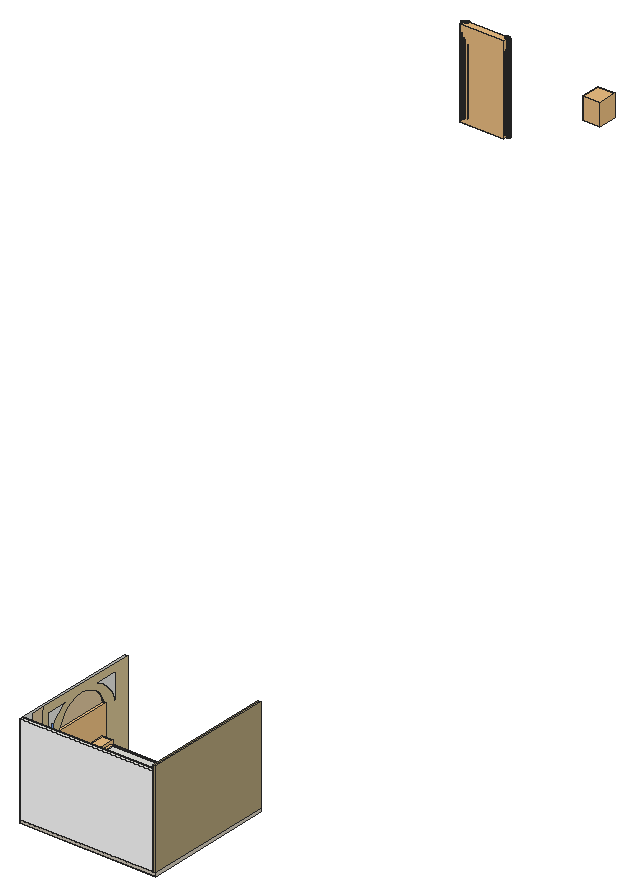
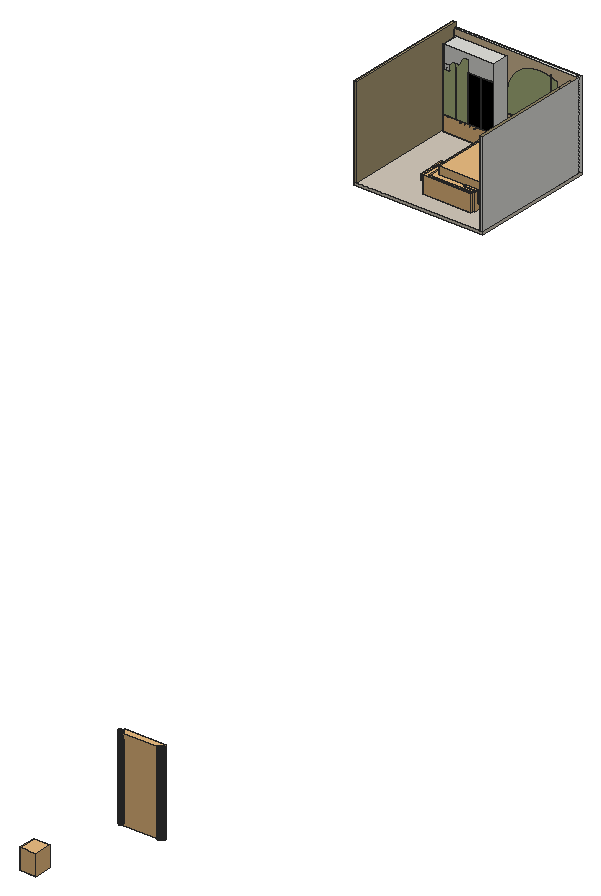
# SketchUp Ruby script. Lengths in inches.
U = 1.inch
M = Sketchup.active_model
def pt(a) = Geom::Point3d.new(a.map { |v| v * U })
def face(e, loops, mat)
  f = e.add_face(loops[0].map { |a| pt(a) })
  loops[1..].each { |l| e.add_face(l.map { |a| pt(a) }).erase! }
  f.material = f.back_material = mat if mat
  f
end
# faces: each face lists its corners as indices into pts; further lists are holes
def faces(e, pts, list, mat = nil) = list.each { |f| face(e, (f[0].is_a?(Array) ? f : [f]).map { |l| l.map { |i| pts[i] } }, mat) }
# xy, xz, yz: faces in a plane at the given z, y or x. An outline is a flat list of corners, or four numbers for a rectangle; further outlines are holes
def ring(l) = l.size == 4 ? [[l[0], l[1]], [l[2], l[1]], [l[2], l[3]], [l[0], l[3]]] : l.each_slice(2).to_a
def flat(e, list, mat, &to3) = list.each { |f| face(e, (f[0].is_a?(Array) ? f : [f]).map { |l| ring(l).map { |u, v| to3.(u, v) } }, mat) }
def xy(e, z, list, mat = nil) = flat(e, list, mat) { |x, y| [x, y, z] }
def xz(e, y, list, mat = nil) = flat(e, list, mat) { |x, z| [x, y, z] }
def yz(e, x, list, mat = nil) = flat(e, list, mat) { |y, z| [x, y, z] }
def lines(e, pts, list) = list.each { |a, b| e.add_line(pt(pts[a]), pt(pts[b])) }
# prism: a flat outline (further loops are holes) pulled along v
def prism(e, loops, v, mat = nil)
  f = face(e, loops, mat); d = Geom::Vector3d.new(v.map { |x| x * U })
  f.pushpull(f.normal.samedirection?(d) ? d.length : -d.length)
end
def box(e, o, s, mat = nil) = prism(e, [[o, [o[0] + s[0], o[1], o[2]], [o[0] + s[0], o[1] + s[1], o[2]], [o[0], o[1] + s[1], o[2]]]], [0, 0, s[2]], mat)
def at(x, y, z, deg = 0) = Geom::Transformation.translation(pt([x, y, z])) * Geom::Transformation.rotation(ORIGIN, Z_AXIS, deg.degrees)
def axes(o, x, y, z) = Geom::Transformation.new([*x, 0, *y, 0, *z, 0, *pt(o).to_a, 1])
def part(name) = M.definitions.add(name)
# library, detail: a bought-in or finely detailed component or shape, given as its bounding box
def library(name, o, s) = part(name).tap { |d| box(d.entities, o, s) }
def detail(e, o, s) = box(e.add_group.entities, o, s)
def put(e, d, t, mat = nil) = e.add_instance(d, t).tap { |i| i.material = mat if mat }
def group(e, t, mat = nil) = e.add_group.tap { |g| g.transformation = t; g.material = mat if mat }.entities
root = M.entities
M.materials.add("BACK Wall colour").color = [219, 194, 155]
M.materials.add("CREAM BOARD").color = [211, 192, 145]
M.materials.add("Emissive").color = [255, 225, 187]
M.materials.add("Emissive\#1").color = [255, 255, 255]
M.materials.add("Marble").color = [211, 202, 187]
M.materials.add("Material__1").color = [146, 146, 144]
M.materials.add("Material__10").color = [208, 163, 136]
M.materials.add("Material__11").color = [204, 203, 204]
M.materials.add("Material__2").color = [184, 175, 165]
M.materials.add("Material__3").color = [220, 221, 223]
M.materials.add("Material__4").color = [119, 115, 113]
M.materials.add("Material__5").color = [191, 184, 174]
M.materials.add("Material__6").color = [181, 176, 158]
M.materials.add("Material__8").color = [243, 243, 243]
M.materials.add("Material__9").color = [193, 193, 193]
M.materials.add("[Color A01]").color = [173, 157, 118]
M.materials.add("[Color M07]").color = [57, 57, 57]
M.materials.add("[Translucent Glass Blue]").color = [100, 149, 237]
M.materials["[Translucent Glass Blue]"].alpha = 0.5
M.materials.add("cubod").color = [174, 185, 130]
M.materials.add("mirror").color = [0, 0, 0]
M.materials.add("wire_1").color = [252, 248, 227]
M.materials.add("wire_2").color = [148, 176, 27]
M.materials.add("wire_3").color = [246, 240, 240]
M.materials.add("wire_4").color = [250, 248, 254]
M.materials.add("wire_5").color = [223, 86, 86]
M.materials.add("ไม้ระแนง").color = [255, 207, 170]
c1 = library("Group\#139",[0,-0.62,-0.17],[22.83,25.13,29.45])
c2 = part("Group\#298")
box(c2.entities,[1.18,0.2,0],[0.79,0.19,118.11])
c3 = part("Group\#129")
put(c3.entities,c2,at(1.68,1.9,0,-75.963))
put(c3.entities,c2,at(1.875,1.69,0,-18.991))
put(c3.entities,c2,at(1.72,1.81,0,-56.972))
put(c3.entities,c2,at(1.7,1.85,0,-66.468))
put(c3.entities,c2,at(2.26,1.99,0,94.13))
put(c3.entities,c2,at(1.92,1.68,0,-9.495))
put(c3.entities,c2,at(1.67,2,0,-94.954))
put(c3.entities,c2,at(1.79,1.74,0,-37.981))
put(c3.entities,c2,at(1.7,2.09,0,-113.944))
put(c3.entities,c2,at(1.83,1.71,0,-28.486))
put(c3.entities,c2,at(1.75,1.77,0,-47.477))
put(c3.entities,c2,at(1.68,2.04,0,-104.449))
put(c3.entities,c2,at(1.67,1.95,0,-85.458))
put(c3.entities,c2,at(2.26,1.94,0,84.634))
put(c3.entities,c2,at(1.97,1.67,0))
put(c3.entities,c2,at(2.1875,2.17,0,132.111))
put(c3.entities,c2,at(1.83,2.23,0,-151.926))
put(c3.entities,c2,at(1.75,2.17,0,-132.935))
put(c3.entities,c2,at(1.72,2.13,0,-123.44))
put(c3.entities,c2,at(2.07,2.25,0,160.597))
put(c3.entities,c2,at(2.24,2.09,0,113.12))
put(c3.entities,c2,at(1.92,2.26,0,-170.917))
put(c3.entities,c2,at(2.02,2.26,0,170.093))
put(c3.entities,c2,at(2.11,2.23,0,151.102))
put(c3.entities,c2,at(2.15,2.2,0,141.607))
put(c3.entities,c2,at(2.22,2.13,0,122.616))
put(c3.entities,c2,at(1.875,2.25,0,-161.421))
put(c3.entities,c2,at(2.26,2.04,0,103.625))
put(c3.entities,c2,at(1.79,2.2,0,-142.431))
put(c3.entities,c2,at(1.97,2.27,0,179.588))
put(c3.entities,c2,at(2.0625,1.69,0,18.167))
put(c3.entities,c2,at(2.18,1.77,0,46.653))
put(c3.entities,c2,at(2.25,1.89,0,75.139))
put(c3.entities,c2,at(2.15,1.73,0,37.157))
put(c3.entities,c2,at(2.01,1.68,0,8.671))
put(c3.entities,c2,at(1.92,1.68,0,-10.319))
put(c3.entities,c2,at(1.96,1.67,0,-0.824))
put(c3.entities,c2,at(2.21,1.81,0,56.148))
put(c3.entities,c2,at(1.87,1.69,0,-19.815))
put(c3.entities,c2,at(2.24,1.85,0,65.644))
put(c3.entities,c2,at(2.11,1.71,0,27.662))
c4 = library("Group\#135",[0,0,0],[59.06,10.24,118.11])
c5 = library("Group\#97",[220.84,467.58,-548.74],[526,430.5,273.26])
c6 = library("Group\#96",[16.29,461.76,-808.58],[654.47,563.24,342.1])
c7 = library("Group\#95",[26.77,467.46,-1024.34],[745.52,615.51,329.95])
c8 = library("Group\#94",[-756.47,467.51,-1025.0625],[743.88,650.18,302.68])
c9 = library("Group\#93",[-553.95,461.3125,-816.79],[663.59,570.86,267.16])
c10 = library("Group\#92",[-509.59,467.57,-586.51],[732.34,417.16,267.86])
c11 = library("Group\#91",[-1172.66,2.01,-321.31],[2325.11,593.39,1560.68])
c12 = library("Group\#90",[-1281.34,1.4,-240.6],[2502.68,574.48,1653.76])
c13 = library("Group\#89",[-1090.55,247.54,-372.01],[2133.07,362.54,526.23])
c14 = library("Group\#88",[-193.83,481.2,453.03],[613.57,176.39,387.44])
c15 = library("Group\#87",[-955.4375,-0.64,-1094.53],[1900,840.64,2180.25])
c16 = library("Group\#86",[-945.74,207.56,-988.65],[1854.67,255.51,2057.08])
c17 = library("Group\#85",[-22.63,147.2,1249.93],[883.21,192.64,509.1])
c18 = library("Group\#104",[189.08,342.22,1232.64],[352.42,17.32,353.57])
c19 = library("Group\#105",[41.45,326.8125,1372.4],[357.97,38.32,359.1])
c20 = library("Group\#106",[39.12,326.04,1373.29],[358.62,26.89,359.71])
c21 = library("Group\#98",[-1244.68,656.3,-867.46],[92.26,185.35,88.07])
c22 = library("Group\#99",[-1423.96,598.21,-801.8],[288.83,436.59,261.62])
c23 = library("Group\#100",[-1158.34,656.31,-821.02],[80.76,145.22,75.04])
c24 = library("Group\#101",[-1453.32,0.83,-981.3],[432.86,597.97,432.82])
c25 = library("Group\#102",[-1264.29,598.92,-883.28],[205.66,57.91,141.8])
c26 = library("Group\#103",[202.625,359.35,1362.02],[142.76,55.22,150.9])
c27 = part("bed")
g1 = group(c27.entities,at(-348.48,-2600.07,-0.46))
put(g1,c5,axes([1281.34,1759.03,0.64],[1,0,0],[0,0,1],[0,-1,0]),"Material__1")
put(g1,c6,axes([1281.34,1759.03,0.64],[1,0,0],[0,0,1],[0,-1,0]),"Material__2")
put(g1,c7,axes([1281.34,1759.03,0.64],[1,0,0],[0,0,1],[0,-1,0]),"Material__3")
put(g1,c8,axes([1281.34,1759.03,0.64],[1,0,0],[0,0,1],[0,-1,0]),"Material__2")
put(g1,c9,axes([1281.34,1759.03,0.64],[1,0,0],[0,0,1],[0,-1,0]),"Material__3")
put(g1,c10,axes([1281.34,1759.03,0.64],[1,0,0],[0,0,1],[0,-1,0]),"Material__4")
put(g1,c11,axes([1281.34,1759.03,0.64],[1,0,0],[0,0,1],[0,-1,0]),"Material__2")
put(g1,c12,axes([1281.34,1759.03,0.64],[1,0,0],[0,0,1],[0,-1,0]),"Material__4")
put(g1,c13,axes([1281.34,1759.03,0.64],[1,0,0],[0,0,1],[0,-1,0]),"Material__3")
put(g1,c14,axes([1281.34,1759.03,0.64],[1,0,0],[0,0,1],[0,-1,0]),"Material__5")
put(g1,c15,axes([1281.34,1759.03,0.64],[1,0,0],[0,0,1],[0,-1,0]),"Material__6")
put(g1,c16,axes([1281.34,1759.03,0.64],[1,0,0],[0,0,1],[0,-1,0]),"wire_1")
put(g1,c17,axes([1281.34,1759.03,0.64],[1,0,0],[0,0,1],[0,-1,0]),"Material__6")
g2 = group(g1,at(1281.34,1759.03,0.64),"Material__6")
p = [[51.41,-1680.01,120.74],[789.14,-1719.33,120.75],[51.38,-1719.36,120.79],[51.38,-1680.06,160.45],[788.85,-1679.65,121.17],[789.14,-1679.64,160.07],
  [788.85,-1718.96,160.45],[51.74,-1719.36,160.07]]
faces(g2,p,[[0,1,2],[3,0,2],[0,4,1],[0,3,5],[0,5,4],[6,2,1],[6,7,2],[3,2,7],
  [6,1,4],[6,4,5],[7,5,3],[7,6,5]],"[Color M07]")
g3 = group(g1,at(1281.34,1759.03,0.64),"Material__6")
p = [[788.42,-1678.8,120.79],[827.72,-1336.33,121.1],[827.72,-1678.5,120.76],[788.4,-1336.69,121.17],[788.38,-1336.73,160.09],[788.41,-1678.49,160.09],
  [828.07,-1678.51,160.45],[828.09,-1336.73,160.41]]
faces(g3,p,[[0,1,2],[0,3,1],[0,4,3],[0,5,4],[7,2,1],[7,6,2],[7,1,3],[7,3,4],
  [6,4,5],[6,7,4]],"[Color M07]")
faces(g3,p,[[5,0,2],[5,2,6]],"Material__6")
g4 = group(g1,at(1281.34,1759.03,0.64),"Material__6")
p = [[51.36,-1295.89,160.46],[51.45,-1335.18,120.84],[51.35,-1333.34,160.1],[52.33,-1335.21,158.6],[51.47,-1295.85,120.75],[789.16,-1335.14,120.79],
  [788.81,-1335.18,160.42],[789.15,-1295.51,120.8125],[788.78,-1295.48,160.09]]
faces(g4,p,[[0,1,2],[1,3,2],[4,5,1],[6,1,5],[6,3,1],[0,4,1],[6,7,8],[6,5,7],
  [4,7,5],[4,0,8],[4,8,7],[6,2,3],[2,6,8],[2,8,0]],"[Color M07]")
g5 = group(g1,at(1281.34,1759.03,0.64),"Material__6")
p = [[12.71,-1678.78,120.74],[12.34,-1336.83,160.45],[12.72,-1336.33,121.11],[12.71,-1678.52,160.09],[51.7,-1336.34,121.1],[52.03,-1678.85,120.78],
  [52.03,-1678.82,160.45],[52.06,-1336.72,160.4]]
faces(g5,p,[[0,1,2],[0,3,1],[0,4,5],[0,2,4],[3,0,5],[3,5,6],[7,5,4],[7,6,5],
  [7,2,1],[7,4,2],[6,1,3],[6,7,1]],"[Color M07]")
g6 = group(g1,at(1281.34,1759.03,0.64),"Material__6")
xy(g6,160.97,[[12.77,-1334.88,51.14,-1295.51,11.77,-1296.13],[12.77,-1334.88,51.14,-1334.51,51.14,-1295.51]],"[Color M07]")
p = [[11.77,-1296.13,160.97],[11.86,-1295.16,1.14],[11.8,-1334.85,1.21],[45.68,-1334.49,1.53],[45.32,-1295.17,1.54],[51.14,-1295.51,160.97],
  [12.77,-1334.88,160.97],[51.14,-1334.51,160.97]]
faces(g6,p,[[0,1,2],[3,2,1],[3,1,4],[1,0,5],[1,5,4],[0,2,6],[7,2,3],[7,6,2],
  [7,4,5],[7,3,4]],"[Color M07]")
g7 = group(g1,at(1281.34,1759.03,0.64),"Material__6")
xy(g7,160.97,[[788.98,-1334.51,828.36,-1296.13,789.61,-1295.13],[788.98,-1334.51,828.36,-1333.88,828.36,-1296.13]],"[Color M07]")
p = [[794.82,-1295.53,1.14],[794.46,-1334.78,1.52],[788.98,-1334.51,160.97],[828.27,-1295.17,1.16],[789.61,-1295.13,160.97],[828.34,-1334.85,1.52],
  [828.36,-1296.13,160.97],[828.36,-1333.88,160.97]]
faces(g7,p,[[0,1,2],[3,1,0],[0,2,4],[4,3,0],[3,5,1],[5,3,6],[4,6,3],[5,2,1],
  [5,7,2],[5,6,7]],"[Color M07]")
g8 = group(g1,at(1281.34,1759.03,0.64),"Material__6")
xy(g8,160.97,[[12.14,-1718.67,50.52,-1679.3,11.77,-1680.3],[12.14,-1718.67,51.14,-1718.67,50.52,-1679.3]],"[Color M07]")
p = [[11.77,-1680.3,160.97],[11.8125,-1679.33,1.15],[11.82,-1719.03,1.51],[45.67,-1718.59,1.49],[45.67,-1679.4,1.55],[50.52,-1679.3,160.97],
  [12.14,-1718.67,160.97],[51.14,-1718.67,160.97]]
faces(g8,p,[[0,1,2],[3,2,1],[3,1,4],[1,0,5],[1,5,4],[0,2,6],[7,2,3],[7,6,2],
  [7,4,5],[7,3,4]],"[Color M07]")
g9 = group(g1,at(1281.34,1759.03,0.64),"Material__6")
xy(g9,160.97,[[827.36,-1719.05,827.98,-1679.67,788.98,-1718.67],[788.98,-1718.67,827.98,-1679.67,789.61,-1679.3]],"[Color M07]")
p = [[788.98,-1718.67,160.97],[794.47,-1718.58,1.13],[827.91,-1719.01,1.18],[828.34,-1679.72,1.49],[794.48,-1679.34,1.55],[827.36,-1719.05,160.97],
  [827.98,-1679.67,160.97],[789.61,-1679.3,160.97]]
faces(g9,p,[[0,1,2],[3,2,1],[4,1,0],[3,1,4],[0,2,5],[2,6,5],[2,3,6],[3,7,6],
  [3,4,7],[4,0,7]],"[Color M07]")
g10 = group(c27.entities,at(-528.95,-2575.43,-0.01))
put(g10,c18,axes([1453.32,1733,-0.83],[1,0,0],[0,0,1],[0,-1,0]),"Material__10")
put(g10,c19,axes([1453.32,1733,-0.83],[1,0,0],[0,0,1],[0,-1,0]),"Material__11")
put(g10,c20,axes([1453.32,1733,-0.83],[1,0,0],[0,0,1],[0,-1,0]),"Material__10")
g11 = group(g10,at(1453.32,1733,-0.83),"Material__10")
xy(g11,341.8125,[[398.96,-1586.72,187.8125,-1372.09,331.77,-1230.46],[398.96,-1586.72,331.77,-1230.46,542.92,-1445.09]],"Material__10")
xy(g11,342.21,[[398.96,-1586.72,542.92,-1445.09,187.8125,-1372.09],[542.92,-1445.09,331.77,-1230.46,187.8125,-1372.09]],"Material__10")
p = [[398.96,-1586.72,342.21],[187.8125,-1372.09,341.8125],[398.96,-1586.72,341.8125],[187.8125,-1372.09,342.21],[542.92,-1445.09,342.21],[542.92,-1445.09,341.8125],
  [331.77,-1230.46,341.8125],[331.77,-1230.46,342.21]]
faces(g11,p,[[0,1,2],[1,0,3],[4,2,5],[2,4,0],[4,6,7],[4,5,6],[1,7,6],[1,3,7]],"Material__10")
g12 = group(g10,at(1453.32,1733,-0.83),"Material__10")
p = [[52.72,-1506.35,338.55],[45.44,-1513.52,338.34],[255.83,-1727.375,338.34],[263.11,-1720.21,338.55],[59.99,-1499.2,339.34],[270.375,-1713.06,339.34],
  [67.24,-1492.07,340.6],[277.63,-1705.93,340.6],[74.48,-1484.94,342.23],[284.87,-1698.8,342.23],[81.7,-1477.84,344.15],[292.09,-1691.7,344.15],
  [88.92,-1470.74,346.45],[299.31,-1684.6,346.45],[96.12,-1463.66,349.28],[306.51,-1677.52,349.28],[103.31,-1456.58,352.49],[313.7,-1670.44,352.49],
  [110.49,-1449.52,355.9],[320.88,-1663.38,355.9],[117.66,-1442.47,359.33],[328.05,-1656.33,359.33],[188.98,-1372.29,357.09],[181.87,-1379.29,362.68],
  [392.26,-1593.15,362.65],[399.375,-1586.15,357.09],[124.82,-1435.42,362.6],[335.21,-1649.28,362.6],[131.97,-1428.38,365.54],[342.36,-1642.24,365.53],
  [385.15,-1600.15,366.64],[174.76,-1386.29,366.71],[139.12,-1421.35,367.96],[349.51,-1635.21,367.96],[378.03,-1607.16,369.19],[167.64,-1393.3,369.26],
  [146.25,-1414.33,369.7],[356.64,-1628.19,369.7],[370.9,-1614.16,370.46],[160.51,-1400.3,370.51],[153.39,-1407.32,370.6],[363.78,-1621.17,370.58]]
faces(g12,p,[[0,1,2],[0,2,3],[3,4,0],[3,5,4],[6,4,5],[6,5,7],[7,8,6],[7,9,8],
  [10,8,9],[10,9,11],[11,12,10],[11,13,12],[13,14,12],[13,15,14],[16,14,15],[16,15,17],
  [17,18,16],[17,19,18],[20,18,19],[20,19,21],[22,23,24],[22,24,25],[26,20,21],[26,21,27],
  [27,28,26],[27,29,28],[30,24,23],[30,23,31],[32,28,29],[32,29,33],[34,30,31],[34,31,35],
  [33,36,32],[33,37,36],[35,38,34],[35,39,38],[40,36,37],[40,37,41],[41,39,40],[41,38,39]],"Material__10")
g13 = group(g10,at(1453.32,1733,-0.83),"Material__10")
p = [[53.07,-1506.71,338.02],[45.78,-1513.87,337.94],[256.18,-1727.73,337.94],[263.46,-1720.57,338.02],[60.34,-1499.56,338.62],[270.73,-1713.42,338.62],
  [67.59,-1492.42,339.66],[277.98,-1706.28,339.66],[74.83,-1485.3,341.05],[285.22,-1699.16,341.05],[82.05,-1478.19,342.71],[292.44,-1692.05,342.71],
  [89.27,-1471.1,344.72],[299.66,-1684.95,344.72],[96.47,-1464.01,347.27],[306.86,-1677.87,347.28],[103.66,-1456.9375,350.23],[314.05,-1670.8,350.24],
  [110.84,-1449.875,353.41],[321.23,-1663.73,353.42],[118.01,-1442.82,356.67],[328.4,-1656.68,356.67],[125.17,-1435.78,359.8125],[335.56,-1649.64,359.82],
  [189.33,-1372.65,357.16],[182.22,-1379.65,361.98],[392.61,-1593.51,361.95],[399.72,-1586.51,357.16],[132.32,-1428.74,362.68],[342.71,-1642.6,362.69],
  [385.5,-1600.51,365.3],[175.11,-1386.65,365.375],[139.47,-1421.71,365.125],[349.86,-1635.57,365.13],[146.6,-1414.6875,366.97],[356.99,-1628.55,366.95],
  [378.375,-1607.51,367.34],[167.99,-1393.65,367.42],[153.74,-1407.67,368.07],[364.125,-1621.53,368.01],[371.25,-1614.52,368.19],[160.86,-1400.66,368.27]]
faces(g13,p,[[0,1,2],[0,2,3],[3,4,0],[3,5,4],[6,4,5],[6,5,7],[7,8,6],[7,9,8],
  [10,8,9],[10,9,11],[11,12,10],[11,13,12],[13,14,12],[13,15,14],[15,16,14],[15,17,16],
  [18,16,17],[18,17,19],[19,20,18],[19,21,20],[21,22,20],[21,23,22],[24,25,26],[24,26,27],
  [23,28,22],[23,29,28],[30,26,25],[30,25,31],[32,28,29],[32,29,33],[33,34,32],[33,35,34],
  [36,30,31],[36,31,37],[38,34,35],[38,35,39],[37,40,36],[37,41,40],[39,41,38],[39,40,41]],"Material__10")
g14 = group(g10,at(1453.32,1733,-0.83),"Material__10")
xy(g14,341.8125,[[399.85,-1587.61,187.8125,-1372.09,188.38,-1371.53],[399.85,-1587.61,188.38,-1371.53,400.41,-1587.06]],"Material__10")
xy(g14,357.01,[[400.31,-1587.16,188.38,-1371.53,188.28,-1371.63],[400.31,-1587.16,400.41,-1587.06,188.38,-1371.53]],"Material__10")
p = [[188.24,-1371.67,344.34],[187.8125,-1372.09,341.8125],[399.85,-1587.61,341.8125],[400.27,-1587.2,344.34],[400.83,-1586.64,344.34],[400.41,-1587.06,341.8125],
  [188.38,-1371.53,341.8125],[188.8,-1371.12,344.34],[271.2,-1455.72,347.08],[329.7,-1515.2,346.88],[400.41,-1587.06,347.24],[400.97,-1586.51,349.41],
  [188.93,-1370.99,346.88],[377.41,-1562.57,346.88],[188.36,-1371.55,346.79],[235.46,-1419.47,354.48],[188.28,-1371.63,357.01],[188.9,-1371.02,354.48],
  [188.89,-1371.03,350.78],[188.93,-1370.99,349.41],[353.28,-1539.17,349.41],[299.14,-1484.21,351.8],[259.01,-1443.43,351.94],[400.36,-1587.11,351.94],
  [400.92,-1586.56,351.94],[400.93,-1586.54,354.48],[400.37,-1587.1,354.48],[400.31,-1587.16,357.01],[400.41,-1587.06,357.01],[188.38,-1371.53,357.01]]
faces(g14,p,[[0,1,2],[2,3,0],[4,2,5],[4,3,2],[4,5,6],[4,6,7],[1,7,6],[1,0,7],
  [3,8,0],[3,9,8],[3,10,9],[4,10,3],[10,4,11],[12,4,7],[4,12,13],[11,4,13],
  [14,0,8],[12,0,14],[12,7,0],[8,15,14],[14,15,16],[14,16,17],[14,17,18],[18,19,14],
  [19,12,14],[10,20,9],[12,11,13],[12,19,11],[21,9,20],[22,9,21],[22,8,9],[8,22,15],
  [23,20,10],[10,24,23],[10,11,24],[23,21,20],[19,24,11],[19,25,24],[19,18,25],[25,18,17],
  [26,22,21],[23,26,21],[22,26,15],[23,25,26],[23,24,25],[15,27,16],[27,15,26],[26,28,27],
  [28,25,29],[26,25,28],[29,25,17],[29,17,16]],"Material__10")
g15 = group(g10,at(1453.32,1733,-0.83),"Material__10")
p = [[399.05,-1588.4,347.87],[398.51,-1588.93,348.09],[187.02,-1372.87,347.87],[280.71,-1469.19,348.09],[399.53,-1587.92,350.23],[281.47,-1468.45,348.92],
  [313.21,-1498.64,354.4],[251.51,-1437.57,349.97],[188.27,-1371.64,354.41],[186.47,-1373.4,348.09],[186.9,-1372.98,350.1875],[304.7,-1492.72,350.1875],
  [305.06,-1492.37,352.25],[398.89,-1588.55,349.93],[257.9375,-1444.48,352.25],[257.58,-1444.82,350.1875],[399.29,-1588.16,352.25],[359.9,-1546.94,352.3],
  [400.3,-1587.17,354.39],[210.82,-1396.58,352.25],[211.79,-1395.625,356.71],[188.23,-1371.68,356.71],[399.84,-1587.62,354.61],[400.35,-1587.12,356.49],
  [188.32,-1371.59,356.49],[400.26,-1587.2,356.71]]
faces(g15,p,[[0,1,2],[3,2,1],[1,0,4],[4,0,2],[2,5,4],[2,6,7],[2,8,6],[2,3,9],
  [2,7,5],[2,9,10],[8,2,10],[1,11,3],[11,1,12],[1,13,12],[1,4,13],[12,3,11],
  [3,12,14],[15,9,3],[3,14,15],[9,15,10],[4,5,7],[13,16,12],[4,16,13],[4,7,17],
  [6,17,7],[18,16,4],[18,4,17],[19,10,15],[19,15,14],[19,20,10],[21,10,20],[10,21,8],
  [22,12,16],[18,22,16],[19,22,20],[22,19,14],[22,14,12],[18,17,6],[22,18,23],[23,18,6],
  [23,6,24],[24,6,8],[24,8,21],[20,22,25],[22,23,25],[25,23,24],[24,20,25],[24,21,20]],"Material__10")
put(g10,c21,axes([1453.32,1733,-0.83],[1,0,0],[0,0,1],[0,-1,0]),"Material__8")
put(g10,c22,axes([1453.32,1733,-0.83],[1,0,0],[0,0,1],[0,-1,0]),"wire_2")
put(g10,c23,axes([1453.32,1733,-0.83],[1,0,0],[0,0,1],[0,-1,0]),"wire_3")
put(g10,c24,axes([1453.32,1733,-0.83],[1,0,0],[0,0,1],[0,-1,0]),"wire_4")
put(g10,c25,axes([1453.32,1733,-0.83],[1,0,0],[0,0,1],[0,-1,0]),"Material__9")
put(g10,c26,axes([1453.32,1733,-0.83],[1,0,0],[0,0,1],[0,-1,0]),"wire_5")
c28 = library("Group\#121",[0,0,0],[71.63,0.32,21.29])
c29 = part("Group\#9")
prism(c29.entities,[[[1.125,0,43.59],[1.125,0,42.2],[1.125,4.02,42.2],[1.125,4.02,1.84],[1.125,3.28,1.84],[1.125,0,1.84],[1.125,0,0],[1.125,4.41,0],[1.125,4.53,0.01],[1.125,4.64,0.03],[1.125,4.76,0.07],[1.125,4.86,0.12],[1.125,4.96,0.1875],[1.125,5.05,0.26],[1.125,5.125,0.35],[1.125,5.19,0.45],[1.125,5.24,0.56],[1.125,5.28,0.67],[1.125,5.3,0.79],[1.125,5.3125,0.9],[1.125,5.3125,42.39],[1.125,5.3,42.54],[1.125,5.28,42.68],[1.125,5.23,42.82],[1.125,5.17,42.95],[1.125,5.1,43.08],[1.125,5,43.19],[1.125,4.9,43.3],[1.125,4.78,43.39],[1.125,4.66,43.46],[1.125,4.52,43.52],[1.125,4.38,43.56],[1.125,4.24,43.59]]],[-0.5625,0,0])
c30 = library("Group\#232",[0,0,0],[7.29,6.21,8.93])
c31 = library("Group\#117",[0,0,-15.125],[6.625,128.97,92.32])
xy(root,4,[[584.79,4,584.79,176.875,588.79,176.875,588.79,138.88,585.35,138.88,585.35,59.66,588.79,59.66,588.79,4],[588.79,4,608.79,15.125],[608.79,4,616.04,15.125]])
xy(root,6.25,[[688.79,27,760.79,27.75]])
xy(root,6.34,[[588.79,15.125,589.4375,16],[589.4375,15.125,615.39,16],[615.39,15.125,616.04,16]])
xy(root,15.87,[[614.17,15.625,615.39,16]],"cubod")
xy(root,15.88,[[589.4375,15.625,613.52,16]],"cubod")
xy(root,16.03,[[614.17,15.625,615.39,16]],"cubod")
xy(root,16.04,[[589.4375,15.625,613.52,16]],"cubod")
xy(root,25.87,[[614.17,15.625,615.39,16]],"cubod")
xy(root,25.88,[[589.4375,15.625,613.52,16]],"cubod")
xy(root,26.03,[[614.17,15.625,615.39,16]],"cubod")
xy(root,26.04,[[589.4375,15.625,613.52,16]],"cubod")
xy(root,28,[[688.79,27,760.79,27.75]])
xy(root,28.31,[[688.79,27,706.63,27.75],[706.79,27,724.63,27.75],[724.79,27,742.63,27.75],[742.79,27,760.79,27.75]])
xz(root,4,[[584.79,4,588.79,126.48],[588.79,4,616.04,4,616.04,34.39,615.39,34.39,615.39,34.38,614.17,34.38,613.52,34.39,589.4375,34.39,589.4375,64,588.79,64]])
xz(root,15.125,[[588.79,4,616.04,6.34]])
xz(root,15.625,[[614.17,15.87,613.52,15.88,589.4375,15.88,589.4375,16.04,613.52,16.04,614.17,16.03,615.39,16.03,615.39,15.87],[614.17,25.87,613.52,25.88,589.4375,25.88,589.4375,26.04,613.52,26.04,614.17,26.03,615.39,26.03,615.39,25.87]],"cubod")
xz(root,16,[[[588.79,6.34,588.79,124,589.4375,124,589.4375,94.39,615.39,94.39,615.39,124,616.04,124,616.04,6.34,615.39,6.34,615.39,33.99,614.17,33.99,613.52,34,589.4375,34,589.4375,6.34],[614.17,34.38,615.39,34.38,615.39,64,589.4375,64,589.4375,34.39,613.52,34.39],[589.4375,64.39,615.39,94]]],"[Translucent Glass Blue]")
xz(root,16,[[589.4375,6.34,589.4375,15.88,613.52,15.88,614.17,15.87,615.39,15.87,615.39,6.34],[614.17,16.03,613.52,16.04,589.4375,16.04,589.4375,25.88,613.52,25.88,614.17,25.87,615.39,25.87,615.39,16.03],[614.17,26.03,613.52,26.04,589.4375,26.04,589.4375,34,613.52,34,614.17,33.99,615.39,33.99,615.39,26.03]],"cubod")
xz(root,27,[[688.79,6.25,760.79,28],[688.79,28,706.79,28.31],[706.79,28,724.79,28.31],[724.79,28,742.79,28.31],[742.79,28,760.79,28.31],
  [688.79,28.31,706.63,93.69],[706.63,28.31,706.79,93.69],[706.79,28.31,724.63,93.69],[724.63,28.31,724.79,93.69],[724.79,28.31,742.63,93.69],
  [742.63,28.31,742.79,93.69],[742.79,28.31,760.79,93.69]])
xz(root,27.75,[[688.79,6.25,760.79,28]])
xz(root,27.75,[[724.79,28.31,724.79,109.92,725.14,109.99,727.86,109.83,730.44,108.97,732.71,107.46,734.52,105.42,735.74,102.99,736.29,100.32,736.125,97.6,735.26,95.01,736.64,96.79,738.42,98.14,740.5,98.99,742.63,99.26,742.63,28.31],[742.79,28.31,742.79,99.26,744.95,98.97,747.02,98.1,748.79,96.73,750.15,94.9375,750.99,92.86,751.28,90.64,750.97,88.41,750.1,86.35,760.79,86.35,760.79,28.31]],"cubod")
xz(root,27.75,[[688.79,28.31,706.63,93.69],[706.79,28.31,724.63,93.69]],"mirror")
xz(root,138.88,[[587.07,4,588.79,71.16]])
xz(root,138.88,[[585.35,4,587.07,71.16]],"Emissive")
xz(root,176.875,[[584.79,4,588.79,126.48]])
yz(root,584.79,[[4,4,176.875,126.48]])
yz(root,585.35,[[59.66,4,138.88,4,138.88,76.51,137.54,86.73,133.59,96.27,127.31,104.45,119.125,110.73,109.59,114.68,99.36,116.03,89.14,114.68,79.6,110.73,71.42,104.45,65.14,96.27,61.19,86.73,59.84,76.51]],"BACK Wall colour")
yz(root,588.79,[[4,4,15.125,4,15.125,6.34,16,6.34,16,34,4,34]])
yz(root,588.79,[[15.125,4,34.2,4,34.2,126.48,16,126.48,16,6.34,15.125,6.34]],"BACK Wall colour")
yz(root,588.79,[[[34.2,4,59.66,4,59.84,76.51,61.19,86.73,65.14,96.27,71.42,104.45,79.6,110.73,89.14,114.68,99.36,116.03,109.59,114.68,119.125,110.73,127.31,104.45,133.59,96.27,137.54,86.73,138.88,76.51,138.88,4,176.875,4,176.875,126.48,34.2,126.48],[41.03,64,41.03,117.17,77.31,117.17,76.16,116.7,71.11,114.29,66.32,111.41,61.83,108.07,57.69,104.3125,53.94,100.16,50.61,95.67,47.74,90.87,45.36,85.81,43.48,80.54,42.12,75.12,41.3,69.59],[157.17,64,157.05,69.59,156.37,75.14,155.12,80.59,153.33,85.89,151,90.98,148.18,95.8,144.87,100.31,141.13,104.47,136.98,108.22,132.47,111.53,127.65,114.37,122.57,116.7,121.42,117.17,157.17,117.17]]],"CREAM BOARD")
yz(root,589.4375,[[15.625,15.88,16,16.04],[15.625,25.88,16,26.04]],"cubod")
yz(root,615.39,[[15.625,15.87,16,16.03],[15.625,25.87,16,26.03]],"cubod")
yz(root,616.04,[[4,4,15.125,4,15.125,6.34,16,6.34,16,34.31,4,34.31]])
yz(root,688.79,[[27,6.25,27.75,28],[27,28.31,27.75,34.81]])
yz(root,706.63,[[27,28.31,27.75,93.69]])
yz(root,706.79,[[27,28.31,27.75,93.69]])
yz(root,724.63,[[27,28.31,27.75,93.69]])
yz(root,724.79,[[27,28.31,27.75,93.69]])
yz(root,742.63,[[27,28.31,27.75,93.69]])
yz(root,742.79,[[27,28.31,27.75,93.69]])
yz(root,760.79,[[27,6.25,27.75,28],[27,28.31,27.75,118]])
p = [[585.35,59.84,76.51],[587.07,59.84,76.51],[587.07,59.66,4],[585.35,59.66,4],[588.79,59.66,4],[588.79,59.84,76.51],
  [614.17,16,15.87],[613.52,16,15.88],[613.52,15.625,15.88],[614.17,15.625,15.87],[613.52,16,16.04],[614.17,16,16.03],
  [614.17,15.625,16.03],[613.52,15.625,16.04],[614.17,16,25.87],[613.52,16,25.88],[613.52,15.625,25.88],[614.17,15.625,25.87],
  [613.52,16,26.04],[614.17,16,26.03],[614.17,15.625,26.03],[613.52,15.625,26.04]]
faces(root,p,[[0,1,2,3]],"Emissive")
faces(root,p,[[4,2,1,5]])
faces(root,p,[[6,7,8,9],[10,11,12,13],[14,15,16,17],[18,19,20,21]],"cubod")
put(root,c1,at(81.78,1580.25,-18.84))
g16 = group(root,at(584.79,168,0,-90),"Marble")
xy(g16,0,[[-8.875,0,168,184]])
xy(g16,4,[[-8.875,0,168,184]],"Marble")
xz(g16,0,[[-8.875,0,168,4]])
xz(g16,184,[[-8.875,0,168,4]])
yz(g16,-8.875,[[0,0,184,4]])
yz(g16,168,[[0,0,184,4]])
g17 = group(root,at(66.81,1481.11,0,180),"ไม้ระแนง")
put(g17,c3,axes([3.13,0,0],[1.41,0,0],[0,1.41,0],[0,0,1]))
g18 = group(g17,at(0,3.17,0))
put(g18,c2,at(1.68,1.9,0,-75.963))
put(g18,c2,at(1.875,1.69,0,-18.991))
put(g18,c2,at(1.72,1.81,0,-56.972))
put(g18,c2,at(1.7,1.85,0,-66.468))
put(g18,c2,at(2.26,1.99,0,94.13))
put(g18,c2,at(1.92,1.68,0,-9.495))
put(g18,c2,at(1.67,2,0,-94.954))
put(g18,c2,at(1.79,1.74,0,-37.981))
put(g18,c2,at(1.7,2.09,0,-113.944))
put(g18,c2,at(1.83,1.71,0,-28.486))
put(g18,c2,at(1.75,1.77,0,-47.477))
put(g18,c2,at(1.68,2.04,0,-104.449))
put(g18,c2,at(1.67,1.95,0,-85.458))
put(g18,c2,at(2.26,1.94,0,84.634))
put(g18,c2,at(1.97,1.67,0))
put(g18,c2,at(2.1875,2.17,0,132.111))
put(g18,c2,at(1.83,2.23,0,-151.926))
put(g18,c2,at(1.75,2.17,0,-132.935))
put(g18,c2,at(1.72,2.13,0,-123.44))
put(g18,c2,at(2.07,2.25,0,160.597))
put(g18,c2,at(2.24,2.09,0,113.12))
put(g18,c2,at(1.92,2.26,0,-170.917))
put(g18,c2,at(2.02,2.26,0,170.093))
put(g18,c2,at(2.11,2.23,0,151.102))
put(g18,c2,at(2.15,2.2,0,141.607))
put(g18,c2,at(2.22,2.13,0,122.616))
put(g18,c2,at(1.875,2.25,0,-161.421))
put(g18,c2,at(2.26,2.04,0,103.625))
put(g18,c2,at(1.79,2.2,0,-142.431))
put(g18,c2,at(1.97,2.27,0,179.588))
put(g18,c2,at(2.0625,1.69,0,18.167))
put(g18,c2,at(2.18,1.77,0,46.653))
put(g18,c2,at(2.25,1.89,0,75.139))
put(g18,c2,at(2.15,1.73,0,37.157))
put(g18,c2,at(2.01,1.68,0,8.671))
put(g18,c2,at(1.92,1.68,0,-10.319))
put(g18,c2,at(1.96,1.67,0,-0.824))
put(g18,c2,at(2.21,1.81,0,56.148))
put(g18,c2,at(1.87,1.69,0,-19.815))
put(g18,c2,at(2.24,1.85,0,65.644))
put(g18,c2,at(2.11,1.71,0,27.662))
g19 = group(root,at(0,1481.11,0),"ไม้ระแนง")
put(g19,c3,axes([3.13,0,0],[1.41,0,0],[0,-1.41,0],[0,0,1]))
g20 = group(g19,at(0,-3.17,0))
put(g20,c2,axes([1.68,-1.9,0],[0.24255,0.97014,0],[0.97014,-0.24255,0],[0,0,1]))
put(g20,c2,axes([1.875,-1.69,0],[0.94557,0.32542,0],[0.32542,-0.94557,0],[0,0,1]))
put(g20,c2,axes([1.72,-1.81,0],[0.54505,0.83841,0],[0.83841,-0.54505,0],[0,0,1]))
put(g20,c2,axes([1.7,-1.85,0],[0.39927,0.91683,0],[0.91683,-0.39927,0],[0,0,1]))
put(g20,c2,axes([2.26,-1.99,0],[-0.07201,-0.9974,0],[-0.9974,0.07201,0],[0,0,1]))
put(g20,c2,axes([1.92,-1.68,0],[0.9863,0.16497,0],[0.16497,-0.9863,0],[0,0,1]))
put(g20,c2,axes([1.67,-2,0],[-0.08635,0.99626,0],[0.99626,0.08635,0],[0,0,1]))
put(g20,c2,axes([1.79,-1.74,0],[0.78821,0.61541,0],[0.61541,-0.78821,0],[0,0,1]))
put(g20,c2,axes([1.7,-2.09,0],[-0.40585,0.91394,0],[0.91394,0.40585,0],[0,0,1]))
put(g20,c2,axes([1.83,-1.71,0],[0.87893,0.47695,0],[0.47695,-0.87893,0],[0,0,1]))
put(g20,c2,axes([1.75,-1.77,0],[0.67589,0.737,0],[0.737,-0.67589,0],[0,0,1]))
put(g20,c2,axes([1.68,-2.04,0],[-0.24952,0.96837,0],[0.96837,0.24952,0],[0,0,1]))
put(g20,c2,axes([1.67,-1.95,0],[0.07918,0.99686,0],[0.99686,-0.07918,0],[0,0,1]))
put(g20,c2,axes([2.26,-1.94,0],[0.09351,-0.99562,0],[-0.99562,-0.09351,0],[0,0,1]))
put(g20,c2,axes([1.97,-1.67,0],[1,0,0],[0,-1,0],[0,0,1]))
put(g20,c2,axes([2.1875,-2.17,0],[-0.67057,-0.74185,0],[-0.74185,0.67057,0],[0,0,1]))
put(g20,c2,axes([1.83,-2.23,0],[-0.88234,0.47061,0],[0.47061,0.88234,0],[0,0,1]))
g21 = group(g20,at(1.75,-2.17,0))
prism(g21,[[[-1.2,1.58,0],[-0.66,1,0],[-0.52,1.13,0],[-1.05,1.71,0]]],[0,0,118.11])
put(g20,c2,axes([1.72,-2.13,0],[-0.55106,0.83447,0],[0.83447,0.55106,0],[0,0,1]))
put(g20,c2,axes([2.07,-2.25,0],[-0.94321,-0.33221,0],[-0.33221,0.94321,0],[0,0,1]))
put(g20,c2,axes([2.24,-2.09,0],[-0.39266,-0.91968,0],[-0.91968,0.39266,0],[0,0,1]))
put(g20,c2,axes([1.92,-2.26,0],[-0.98746,0.15787,0],[0.15787,0.98746,0],[0,0,1]))
put(g20,c2,axes([2.02,-2.26,0],[-0.98509,-0.17206,0],[-0.17206,0.98509,0],[0,0,1]))
put(g20,c2,axes([2.11,-2.23,0],[-0.87548,-0.48325,0],[-0.48325,0.87548,0],[0,0,1]))
put(g20,c2,axes([2.15,-2.2,0],[-0.78376,-0.62106,0],[-0.62106,0.78376,0],[0,0,1]))
put(g20,c2,axes([2.22,-2.13,0],[-0.539,-0.8423,0],[-0.8423,0.539,0],[0,0,1]))
put(g20,c2,axes([1.875,-2.25,0],[-0.94789,0.31861,0],[0.31861,0.94789,0],[0,0,1]))
put(g20,c2,axes([2.26,-2.04,0],[-0.23557,-0.97186,0],[-0.97186,0.23557,0],[0,0,1]))
put(g20,c2,axes([1.79,-2.2,0],[-0.79261,0.60972,0],[0.60972,0.79261,0],[0,0,1]))
put(g20,c2,axes([1.97,-2.27,0],[-0.99997,-0.00719,0],[-0.00719,0.99997,0],[0,0,1]))
put(g20,c2,axes([2.0625,-1.69,0],[0.95015,-0.31178,0],[-0.31178,-0.95015,0],[0,0,1]))
put(g20,c2,axes([2.18,-1.77,0],[0.68642,-0.72721,0],[-0.72721,-0.68642,0],[0,0,1]))
put(g20,c2,axes([2.25,-1.89,0],[0.25648,-0.96655,0],[-0.96655,-0.25648,0],[0,0,1]))
put(g20,c2,axes([2.15,-1.73,0],[0.79698,-0.60401,0],[-0.60401,-0.79698,0],[0,0,1]))
put(g20,c2,axes([2.01,-1.68,0],[0.98857,-0.15077,0],[-0.15077,-0.98857,0],[0,0,1]))
put(g20,c2,axes([1.92,-1.68,0],[0.98382,0.17914,0],[0.17914,-0.98382,0],[0,0,1]))
put(g20,c2,axes([1.96,-1.67,0],[0.9999,0.01438,0],[0.01438,-0.9999,0],[0,0,1]))
put(g20,c2,axes([2.21,-1.81,0],[0.55705,-0.83048,0],[-0.83048,-0.55705,0],[0,0,1]))
put(g20,c2,axes([1.87,-1.69,0],[0.94079,0.33898,0],[0.33898,-0.94079,0],[0,0,1]))
put(g20,c2,axes([2.24,-1.85,0],[0.41241,-0.911,0],[-0.911,-0.41241,0],[0,0,1]))
put(g20,c2,axes([2.11,-1.71,0],[0.8857,-0.46426,0],[-0.46426,-0.8857,0],[0,0,1]))
put(root,c4,at(62.73,1480.08,0,180))
g22 = group(root,at(764.79,12,4),"[Color A01]")
box(g22,[0,-12,0],[4,176.875,129.27])
g23 = group(root,at(688.79,4,4))
prism(g23,[[[0,0,0],[0,0,114],[0,23,114],[0,23,2.25],[0,22.375,2.25],[0,22.375,0]]],[72,0,0])
g24 = group(root,at(584.79,0,4))
xy(g24,0,[[0,0,180,4]])
xy(g24,122.48,[[0,0,180,4]])
xz(g24,0,[[0,0,180,122.48]],"Emissive\#1")
xz(g24,1.3125,[[31.25,39.44,31.25,105.25,38.41,108.86,46.08,111.22,54.02,112.28,62.04,111.99,69.89,110.375,77.37,107.47,84.26,103.36,90.36,98.17,95.52,92.03,99.58,85.11,102.43,77.62,104,69.75,104,39.44]],"cubod")
xz(g24,4,[[[0,0,180,122.48],[31.25,39.44,104,39.44,104,69.75,102.43,77.62,99.58,85.11,95.52,92.03,90.36,98.17,84.26,103.36,77.37,107.47,69.89,110.375,62.04,111.99,54.02,112.28,46.08,111.22,38.41,108.86,31.25,105.25]]],"BACK Wall colour")
yz(g24,0,[[0,0,4,122.48]])
yz(g24,180,[[0,0,4,122.48]])
p = [[104,4,69.75],[104,1.3125,69.75],[31.25,4,39.44],[31.25,1.3125,39.44],[31.25,4,105.25],[31.25,1.3125,105.25],
  [104,4,39.44],[104,1.3125,39.44]]
lines(g24,p,[[0,1],[2,3],[4,5],[6,7]])
put(root,c27,axes([598.08,60.74,4.28],[0,0.04161,-0.00012],[-0.04161,0,0],[0,0.00012,0.04161]))
put(root,c28,at(689.16,27.75,6.25))
put(root,c29,axes([599.85,16,14.9375],[0,0,-0.7245],[0,0.09734,0],[0.15972,0,0]))
put(root,c30,at(56.57,1477.15,19.68,180))
put(root,c29,axes([599.85,16,24.875],[0,0,-0.7245],[0,0.09734,0],[0.15972,0,0]))
put(root,c29,axes([736.6875,27.75,24.86],[0,0,1],[0,0.1379,0],[-0.52886,0,0]))
put(root,c31,axes([585.35,60.61,39.73],[0.60694,0,0],[0,0.60694,0],[0,0,0.60694]))
put(root,c29,axes([599.85,16,32.75],[0,0,-0.7245],[0,0.09734,0],[0.15972,0,0]))
